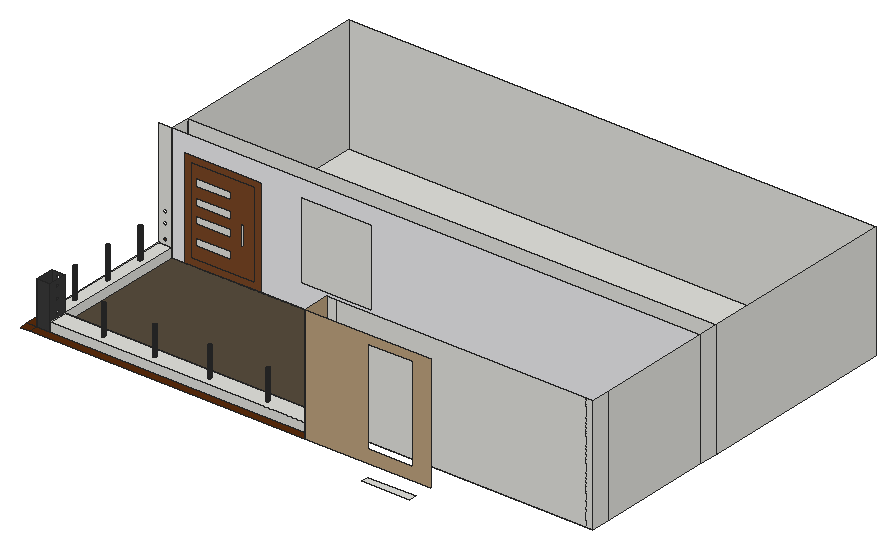
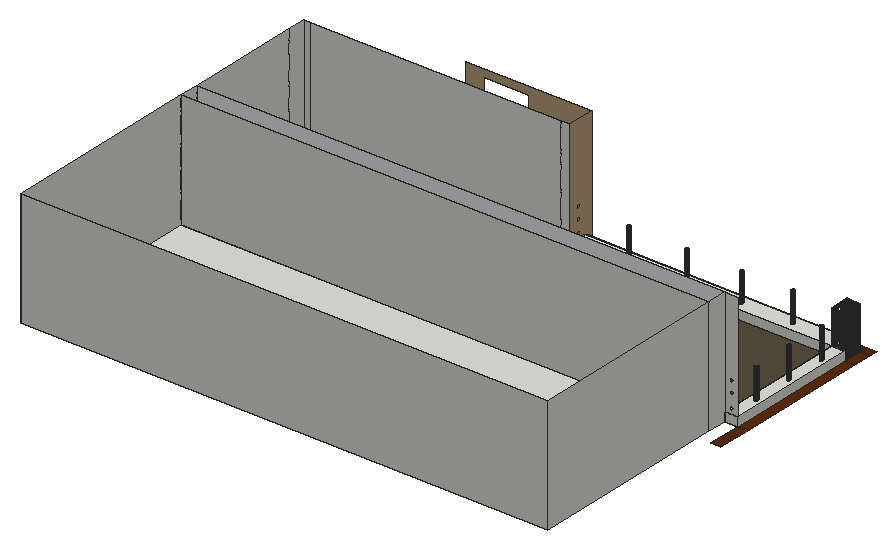
# SketchUp Ruby script. Lengths in inches.
U = 1.inch
M = Sketchup.active_model
def pt(a) = Geom::Point3d.new(a.map { |v| v * U })
def face(e, loops, mat)
  f = e.add_face(loops[0].map { |a| pt(a) })
  loops[1..].each { |l| e.add_face(l.map { |a| pt(a) }).erase! }
  f.material = f.back_material = mat if mat
  f
end
# faces: each face lists its corners as indices into pts; further lists are holes
def faces(e, pts, list, mat = nil) = list.each { |f| face(e, (f[0].is_a?(Array) ? f : [f]).map { |l| l.map { |i| pts[i] } }, mat) }
# xy, xz, yz: faces in a plane at the given z, y or x. An outline is a flat list of corners, or four numbers for a rectangle; further outlines are holes
def ring(l) = l.size == 4 ? [[l[0], l[1]], [l[2], l[1]], [l[2], l[3]], [l[0], l[3]]] : l.each_slice(2).to_a
def flat(e, list, mat, &to3) = list.each { |f| face(e, (f[0].is_a?(Array) ? f : [f]).map { |l| ring(l).map { |u, v| to3.(u, v) } }, mat) }
def xy(e, z, list, mat = nil) = flat(e, list, mat) { |x, y| [x, y, z] }
def xz(e, y, list, mat = nil) = flat(e, list, mat) { |x, z| [x, y, z] }
def yz(e, x, list, mat = nil) = flat(e, list, mat) { |y, z| [x, y, z] }
def lines(e, pts, list) = list.each { |a, b| e.add_line(pt(pts[a]), pt(pts[b])) }
# prism: a flat outline (further loops are holes) pulled along v
def prism(e, loops, v, mat = nil)
  f = face(e, loops, mat); d = Geom::Vector3d.new(v.map { |x| x * U })
  f.pushpull(f.normal.samedirection?(d) ? d.length : -d.length)
end
def box(e, o, s, mat = nil) = prism(e, [[o, [o[0] + s[0], o[1], o[2]], [o[0] + s[0], o[1] + s[1], o[2]], [o[0], o[1] + s[1], o[2]]]], [0, 0, s[2]], mat)
def at(x, y, z, deg = 0) = Geom::Transformation.translation(pt([x, y, z])) * Geom::Transformation.rotation(ORIGIN, Z_AXIS, deg.degrees)
def axes(o, x, y, z) = Geom::Transformation.new([*x, 0, *y, 0, *z, 0, *pt(o).to_a, 1])
def part(name) = M.definitions.add(name)
# library, detail: a bought-in or finely detailed component or shape, given as its bounding box
def library(name, o, s) = part(name).tap { |d| box(d.entities, o, s) }
def detail(e, o, s) = box(e.add_group.entities, o, s)
def put(e, d, t, mat = nil) = e.add_instance(d, t).tap { |i| i.material = mat if mat }
def group(e, t, mat = nil) = e.add_group.tap { |g| g.transformation = t; g.material = mat if mat }.entities
root = M.entities
M.materials.add("[0035_Tan]").color = [188, 161, 125]
M.materials.add("[0043_SaddleBrown]").color = [91, 44, 12]
M.materials.add("[Blinds Vertical Pattern]").color = [237, 237, 239]
M.materials.add("[Carpet Diamond Olive]").color = [87, 77, 61]
M.materials.add("[Color M07]").color = [58, 58, 58]
M.materials.add("[Wood Veneer 01]").color = [120, 70, 37]
xy(root,746.5625,[[378.18,386.34,421.12,393.34]])
xy(root,757.5,[[73.92,401.01,85.98,418.04],[85.98,401.01,320.99,418.04],[73.92,418.04,85.98,538.2],[85.98,538.2,560.26,556.28],[85.98,556.28,560.26,737.09]])
xy(root,757.5,[[65.42,393.34,73.92,401.01],[73.92,393.34,320.99,401.01],[65.42,401.01,73.92,418.04],[65.42,418.04,73.92,538.2],[65.42,538.2,73.92,568.32]],"[0043_SaddleBrown]")
xy(root,757.5,[[85.98,418.04,560.26,538.2]],"[Carpet Diamond Olive]")
xy(root,765.5625,[[[85.98,401.01,320.99,418.04],[127.44,407.81,127.05,407.86,126.69,408.01,126.38,408.25,126.14,408.56,125.99,408.92,125.94,409.31,125.99,409.7,126.14,410.06,126.38,410.37,126.69,410.61,127.05,410.76,127.44,410.81,127.83,410.76,128.19,410.61,128.5,410.37,128.74,410.06,128.89,409.7,128.94,409.31,128.89,408.92,128.74,408.56,128.5,408.25,128.19,408.01,127.83,407.86],[275.5,407.81,275.12,407.86,274.75,408.01,274.44,408.25,274.21,408.56,274.06,408.92,274,409.31,274.06,409.7,274.21,410.06,274.44,410.37,274.75,410.61,275.12,410.76,275.5,410.81,275.89,410.76,276.25,410.61,276.57,410.37,276.8,410.06,276.95,409.7,277,409.31,276.95,408.92,276.8,408.56,276.57,408.25,276.25,408.01,275.89,407.86],[173.82,407.81,173.43,407.86,173.07,408.01,172.76,408.25,172.52,408.56,172.37,408.92,172.32,409.31,172.37,409.7,172.52,410.06,172.76,410.37,173.07,410.61,173.43,410.76,173.82,410.81,174.21,410.76,174.57,410.61,174.88,410.37,175.12,410.06,175.27,409.7,175.32,409.31,175.27,408.92,175.12,408.56,174.88,408.25,174.57,408.01,174.21,407.86],[223,407.81,222.62,407.86,222.25,408.01,221.94,408.25,221.71,408.56,221.56,408.92,221.5,409.31,221.56,409.7,221.71,410.06,221.94,410.37,222.25,410.61,222.62,410.76,223,410.81,223.39,410.76,223.75,410.61,224.07,410.37,224.3,410.06,224.45,409.7,224.5,409.31,224.45,408.92,224.3,408.56,224.07,408.25,223.75,408.01,223.39,407.86]],[127.44,407.81,127.05,407.86,126.69,408.01,126.38,408.25,126.14,408.56,125.99,408.92,125.94,409.31,125.99,409.7,126.14,410.06,126.38,410.37,126.69,410.61,127.05,410.76,127.44,410.81,127.83,410.76,128.19,410.61,128.5,410.37,128.74,410.06,128.89,409.7,128.94,409.31,128.89,408.92,128.74,408.56,128.5,408.25,128.19,408.01,127.83,407.86],[173.82,407.81,173.43,407.86,173.07,408.01,172.76,408.25,172.52,408.56,172.37,408.92,172.32,409.31,172.37,409.7,172.52,410.06,172.76,410.37,173.07,410.61,173.43,410.76,173.82,410.81,174.21,410.76,174.57,410.61,174.88,410.37,175.12,410.06,175.27,409.7,175.32,409.31,175.27,408.92,175.12,408.56,174.88,408.25,174.57,408.01,174.21,407.86],[223,407.81,222.62,407.86,222.25,408.01,221.94,408.25,221.71,408.56,221.56,408.92,221.5,409.31,221.56,409.7,221.71,410.06,221.94,410.37,222.25,410.61,222.62,410.76,223,410.81,223.39,410.76,223.75,410.61,224.07,410.37,224.3,410.06,224.45,409.7,224.5,409.31,224.45,408.92,224.3,408.56,224.07,408.25,223.75,408.01,223.39,407.86],[275.5,407.81,275.12,407.86,274.75,408.01,274.44,408.25,274.21,408.56,274.06,408.92,274,409.31,274.06,409.7,274.21,410.06,274.44,410.37,274.75,410.61,275.12,410.76,275.5,410.81,275.89,410.76,276.25,410.61,276.57,410.37,276.8,410.06,276.95,409.7,277,409.31,276.95,408.92,276.8,408.56,276.57,408.25,276.25,408.01,275.89,407.86],
  [[73.92,418.04,85.98,538.2],[79.17,436.29,78.78,436.34,78.42,436.49,78.11,436.73,77.875,437.04,77.72,437.4,77.67,437.79,77.72,438.18,77.875,438.54,78.11,438.85,78.42,439.09,78.78,439.24,79.17,439.29,79.5625,439.24,79.92,439.09,80.23,438.85,80.47,438.54,80.62,438.18,80.67,437.79,80.62,437.4,80.47,437.04,80.23,436.73,79.92,436.49,79.5625,436.34],[79.17,509.6,78.78,509.65,78.42,509.8,78.11,510.04,77.875,510.35,77.72,510.71,77.67,511.1,77.72,511.49,77.875,511.85,78.11,512.16,78.42,512.4,78.78,512.55,79.17,512.6,79.5625,512.55,79.92,512.4,80.23,512.16,80.47,511.85,80.62,511.49,80.67,511.1,80.62,510.71,80.47,510.35,80.23,510.04,79.92,509.8,79.5625,509.65],[79.17,472.66,78.78,472.72,78.42,472.87,78.11,473.1,77.875,473.41,77.72,473.78,77.67,474.16,77.72,474.55,77.875,474.91,78.11,475.23,78.42,475.46,78.78,475.61,79.17,475.66,79.5625,475.61,79.92,475.46,80.23,475.23,80.47,474.91,80.62,474.55,80.67,474.16,80.62,473.78,80.47,473.41,80.23,473.1,79.92,472.87,79.5625,472.72]],[79.17,436.29,78.78,436.34,78.42,436.49,78.11,436.73,77.875,437.04,77.72,437.4,77.67,437.79,77.72,438.18,77.875,438.54,78.11,438.85,78.42,439.09,78.78,439.24,79.17,439.29,79.5625,439.24,79.92,439.09,80.23,438.85,80.47,438.54,80.62,438.18,80.67,437.79,80.62,437.4,80.47,437.04,80.23,436.73,79.92,436.49,79.5625,436.34],[79.17,472.66,78.78,472.72,78.42,472.87,78.11,473.1,77.875,473.41,77.72,473.78,77.67,474.16,77.72,474.55,77.875,474.91,78.11,475.23,78.42,475.46,78.78,475.61,79.17,475.66,79.5625,475.61,79.92,475.46,80.23,475.23,80.47,474.91,80.62,474.55,80.67,474.16,80.62,473.78,80.47,473.41,80.23,473.1,79.92,472.87,79.5625,472.72],[79.17,509.6,78.78,509.65,78.42,509.8,78.11,510.04,77.875,510.35,77.72,510.71,77.67,511.1,77.72,511.49,77.875,511.85,78.11,512.16,78.42,512.4,78.78,512.55,79.17,512.6,79.5625,512.55,79.92,512.4,80.23,512.16,80.47,511.85,80.62,511.49,80.67,511.1,80.62,510.71,80.47,510.35,80.23,510.04,79.92,509.8,79.5625,509.65]])
xz(root,393.34,[[[320.99,757.5,434.25,861.625],[378.07,769.18,418.25,854.55]]],"[0035_Tan]")
xz(root,401.01,[[85.98,757.5,320.99,765.5625]])
xz(root,401.01,[[73.92,757.5,85.98,796.5]],"[Color M07]")
xz(root,418.04,[[73.92,757.5,85.98,765.5625],[85.98,757.5,320.99,765.5625],[320.99,757.5,329.72,861.625],[329.72,757.5,554.62,861.625],[554.62,757.5,560.26,861.625]])
xz(root,418.04,[[[73.92,765.5625,85.98,796.5],[79.68,781.03,80.13,781.09,80.55,781.27,80.91,781.55,81.19,781.91,81.37,782.33,81.43,782.78,81.37,783.24,81.19,783.66,80.91,784.02,80.55,784.3,80.13,784.47,79.68,784.53,79.22,784.47,78.8,784.3,78.4375,784.02,78.16,783.66,77.99,783.24,77.93,782.78,77.99,782.33,78.16,781.91,78.4375,781.55,78.8,781.27,79.22,781.09],[79.68,768.35,80.13,768.41,80.55,768.58,80.91,768.86,81.19,769.22,81.37,769.64,81.43,770.1,81.37,770.55,81.19,770.97,80.91,771.33,80.55,771.61,80.13,771.79,79.68,771.85,79.22,771.79,78.8,771.61,78.4375,771.33,78.16,770.97,77.99,770.55,77.93,770.1,77.99,769.64,78.16,769.22,78.4375,768.86,78.8,768.58,79.22,768.41],[79.68,790.85,80.13,790.91,80.55,791.08,80.91,791.36,81.19,791.72,81.37,792.14,81.43,792.6,81.37,793.05,81.19,793.47,80.91,793.83,80.55,794.11,80.13,794.29,79.68,794.35,79.22,794.29,78.8,794.11,78.4375,793.83,78.16,793.47,77.99,793.05,77.93,792.6,77.99,792.14,78.16,791.72,78.4375,791.36,78.8,791.08,79.22,790.91]]],"[Color M07]")
xz(root,538.2,[[73.92,757.5,85.98,765.5625],[[73.92,765.5625,85.98,861.625],[79.68,768.35,79.22,768.41,78.8,768.58,78.4375,768.86,78.16,769.22,77.99,769.64,77.93,770.1,77.99,770.55,78.16,770.97,78.4375,771.33,78.8,771.61,79.22,771.79,79.68,771.85,80.13,771.79,80.55,771.61,80.91,771.33,81.19,770.97,81.37,770.55,81.43,770.1,81.37,769.64,81.19,769.22,80.91,768.86,80.55,768.58,80.13,768.41],[79.68,781.03,79.22,781.09,78.8,781.27,78.4375,781.55,78.16,781.91,77.99,782.33,77.93,782.78,77.99,783.24,78.16,783.66,78.4375,784.02,78.8,784.3,79.22,784.47,79.68,784.53,80.13,784.47,80.55,784.3,80.91,784.02,81.19,783.66,81.37,783.24,81.43,782.78,81.37,782.33,81.19,781.91,80.91,781.55,80.55,781.27,80.13,781.09],[79.68,790.85,79.22,790.91,78.8,791.08,78.4375,791.36,78.16,791.72,77.99,792.14,77.93,792.6,77.99,793.05,78.16,793.47,78.4375,793.83,78.8,794.11,79.22,794.29,79.68,794.35,80.13,794.29,80.55,794.11,80.91,793.83,81.19,793.47,81.37,793.05,81.43,792.6,81.37,792.14,81.19,791.72,80.91,791.36,80.55,791.08,80.13,790.91]]])
xz(root,538.2,[[[85.98,757.5,97.43,757.5,97.43,845.625,165.56,845.625,165.56,757.5,560.26,757.5,560.26,861.625,85.98,861.625],[201.38,777.72,265.3,846.97]]],"[Blinds Vertical Pattern]")
xz(root,538.2,[[[97.43,757.5,165.56,845.625],[102.8,762.87,160.18,840.25]],[[102.8,762.87,160.18,840.25],[107.76,822.27,138.82,829.34],[107.76,774.27,138.82,781.34],[107.76,806.52,138.82,813.59],[107.76,792.02,138.82,799.09],[147.39,788.3,150.51,806.24]]],"[Wood Veneer 01]")
xz(root,556.28,[[85.98,757.5,560.26,861.625]])
xz(root,737.09,[[85.98,757.5,560.26,861.625]])
yz(root,73.92,[[418.04,757.5,538.2,765.5625]])
yz(root,73.92,[[401.01,757.5,418.04,796.5]],"[Color M07]")
yz(root,85.98,[[401.01,757.5,418.04,765.5625],[418.04,757.5,538.2,765.5625],[538.2,757.5,556.28,861.625],[556.28,757.5,737.09,861.625]])
yz(root,85.98,[[[401.01,765.5625,418.04,796.5],[408.91,768.38,408.45,768.44,408.03,768.62,407.67,768.9,407.39,769.26,407.22,769.68,407.16,770.13,407.22,770.59,407.39,771.01,407.67,771.37,408.03,771.65,408.45,771.82,408.91,771.88,409.36,771.82,409.78,771.65,410.14,771.37,410.42,771.01,410.6,770.59,410.66,770.13,410.6,769.68,410.42,769.26,410.14,768.9,409.78,768.62,409.36,768.44],[408.91,789.82,408.45,789.88,408.03,790.06,407.67,790.33,407.39,790.7,407.22,791.12,407.16,791.57,407.22,792.02,407.39,792.45,407.67,792.81,408.03,793.09,408.45,793.26,408.91,793.32,409.36,793.26,409.78,793.09,410.14,792.81,410.42,792.45,410.6,792.02,410.66,791.57,410.6,791.12,410.42,790.7,410.14,790.33,409.78,790.06,409.36,789.88],[408.91,779.13,408.45,779.19,408.03,779.37,407.67,779.65,407.39,780.01,407.22,780.43,407.16,780.88,407.22,781.34,407.39,781.76,407.67,782.12,408.03,782.4,408.45,782.57,408.91,782.63,409.36,782.57,409.78,782.4,410.14,782.12,410.42,781.76,410.6,781.34,410.66,780.88,410.6,780.43,410.42,780.01,410.14,779.65,409.78,779.37,409.36,779.19]]],"[Color M07]")
yz(root,320.99,[[401.01,757.5,418.04,765.5625]])
yz(root,320.99,[[[393.34,757.5,393.34,861.625,418.04,861.625,418.04,765.5625,401.01,765.5625,401.01,757.5],[408.91,768.38,409.36,768.44,409.78,768.62,410.14,768.9,410.42,769.26,410.6,769.68,410.66,770.13,410.6,770.59,410.42,771.01,410.14,771.37,409.78,771.65,409.36,771.82,408.91,771.88,408.45,771.82,408.03,771.65,407.67,771.37,407.39,771.01,407.22,770.59,407.16,770.13,407.22,769.68,407.39,769.26,407.67,768.9,408.03,768.62,408.45,768.44],[408.91,789.82,409.36,789.88,409.78,790.06,410.14,790.33,410.42,790.7,410.6,791.12,410.66,791.57,410.6,792.02,410.42,792.45,410.14,792.81,409.78,793.09,409.36,793.26,408.91,793.32,408.45,793.26,408.03,793.09,407.67,792.81,407.39,792.45,407.22,792.02,407.16,791.57,407.22,791.12,407.39,790.7,407.67,790.33,408.03,790.06,408.45,789.88],[408.91,779.13,409.36,779.19,409.78,779.37,410.14,779.65,410.42,780.01,410.6,780.43,410.66,780.88,410.6,781.34,410.42,781.76,410.14,782.12,409.78,782.4,409.36,782.57,408.91,782.63,408.45,782.57,408.03,782.4,407.67,782.12,407.39,781.76,407.22,781.34,407.16,780.88,407.22,780.43,407.39,780.01,407.67,779.65,408.03,779.37,408.45,779.19]]],"[0035_Tan]")
yz(root,560.26,[[418.04,757.5,434.85,861.625],[434.85,757.5,538.2,861.625],[538.2,757.5,556.28,861.625],[556.28,757.5,737.09,861.625]])
p = [[127.05,407.86,765.5625],[127.44,407.81,765.5625],[127.44,407.81,792.02],[127.05,407.86,792.02],[127.83,407.86,765.5625],[127.83,407.86,792.02],
  [173.43,407.86,765.5625],[173.82,407.81,765.5625],[173.82,407.81,791.0625],[173.43,407.86,791.0625],[174.21,407.86,765.5625],[174.21,407.86,791.0625],
  [222.62,407.86,765.5625],[223,407.81,765.5625],[223,407.81,791.57],[222.62,407.86,791.57],[223.39,407.86,765.5625],[223.39,407.86,791.57],
  [275.12,407.86,765.5625],[275.5,407.81,765.5625],[275.5,407.81,791.5625],[275.12,407.86,791.5625],[275.89,407.86,765.5625],[275.89,407.86,791.5625],
  [126.69,408.01,765.5625],[126.69,408.01,792.02],[128.19,408.01,765.5625],[128.19,408.01,792.02],[173.07,408.01,765.5625],[173.07,408.01,791.0625],
  [174.57,408.01,765.5625],[174.57,408.01,791.0625],[222.25,408.01,765.5625],[222.25,408.01,791.57],[223.75,408.01,765.5625],[223.75,408.01,791.57],
  [274.75,408.01,765.5625],[274.75,408.01,791.5625],[276.25,408.01,765.5625],[276.25,408.01,791.5625],[126.38,408.25,765.5625],[126.38,408.25,792.02],
  [128.5,408.25,765.5625],[128.5,408.25,792.02],[172.76,408.25,765.5625],[172.76,408.25,791.0625],[174.88,408.25,765.5625],[174.88,408.25,791.0625],
  [221.94,408.25,765.5625],[221.94,408.25,791.57],[224.07,408.25,765.5625],[224.07,408.25,791.57],[274.44,408.25,765.5625],[274.44,408.25,791.5625],
  [276.57,408.25,765.5625],[276.57,408.25,791.5625],[126.14,408.56,765.5625],[126.14,408.56,792.02],[128.74,408.56,765.5625],[128.74,408.56,792.02],
  [172.52,408.56,765.5625],[172.52,408.56,791.0625],[175.12,408.56,765.5625],[175.12,408.56,791.0625],[221.71,408.56,765.5625],[221.71,408.56,791.57],
  [224.3,408.56,765.5625],[224.3,408.56,791.57],[274.21,408.56,765.5625],[274.21,408.56,791.5625],[276.8,408.56,765.5625],[276.8,408.56,791.5625],
  [125.99,408.92,765.5625],[125.99,408.92,792.02],[128.89,408.92,765.5625],[128.89,408.92,792.02],[172.37,408.92,765.5625],[172.37,408.92,791.0625],
  [175.27,408.92,765.5625],[175.27,408.92,791.0625],[221.56,408.92,765.5625],[221.56,408.92,791.57],[224.45,408.92,765.5625],[224.45,408.92,791.57],
  [274.06,408.92,765.5625],[274.06,408.92,791.5625],[276.95,408.92,765.5625],[276.95,408.92,791.5625],[125.94,409.31,765.5625],[125.94,409.31,792.02],
  [128.94,409.31,765.5625],[128.94,409.31,792.02],[172.32,409.31,765.5625],[172.32,409.31,791.0625],[175.32,409.31,765.5625],[175.32,409.31,791.0625],
  [221.5,409.31,765.5625],[221.5,409.31,791.57],[224.5,409.31,765.5625],[224.5,409.31,791.57],[274,409.31,765.5625],[274,409.31,791.5625],
  [277,409.31,765.5625],[277,409.31,791.5625],[125.99,409.7,765.5625],[125.99,409.7,792.02],[128.89,409.7,765.5625],[128.89,409.7,792.02],
  [172.37,409.7,765.5625],[172.37,409.7,791.0625],[175.27,409.7,765.5625],[175.27,409.7,791.0625],[221.56,409.7,765.5625],[221.56,409.7,791.57],
  [224.45,409.7,765.5625],[224.45,409.7,791.57],[274.06,409.7,765.5625],[274.06,409.7,791.5625],[276.95,409.7,765.5625],[276.95,409.7,791.5625],
  [126.14,410.06,765.5625],[126.14,410.06,792.02],[128.74,410.06,765.5625],[128.74,410.06,792.02],[172.52,410.06,765.5625],[172.52,410.06,791.0625],
  [175.12,410.06,765.5625],[175.12,410.06,791.0625],[221.71,410.06,765.5625],[221.71,410.06,791.57],[224.3,410.06,765.5625],[224.3,410.06,791.57],
  [274.21,410.06,765.5625],[274.21,410.06,791.5625],[276.8,410.06,765.5625],[276.8,410.06,791.5625],[126.38,410.37,765.5625],[126.38,410.37,792.02],
  [128.5,410.37,765.5625],[128.5,410.37,792.02],[172.76,410.37,765.5625],[172.76,410.37,791.0625],[174.88,410.37,765.5625],[174.88,410.37,791.0625],
  [221.94,410.37,765.5625],[221.94,410.37,791.57],[224.07,410.37,765.5625],[224.07,410.37,791.57],[274.44,410.37,765.5625],[274.44,410.37,791.5625],
  [276.57,410.37,765.5625],[276.57,410.37,791.5625],[126.69,410.61,765.5625],[126.68,410.6,792.02],[126.69,410.61,792.02],[128.19,410.61,765.5625],
  [128.19,410.61,792.02],[128.2,410.6,792.02],[173.07,410.61,765.5625],[173.07,410.61,791.0625],[174.57,410.61,765.5625],[174.57,410.61,791.0625],
  [222.25,410.61,765.5625],[222.25,410.61,791.57],[223.75,410.61,765.5625],[223.75,410.61,791.57],[274.75,410.61,765.5625],[274.75,410.61,791.5625],
  [276.25,410.61,765.5625],[276.25,410.61,791.5625],[127.05,410.76,765.5625],[127.05,410.76,792.02],[127.83,410.76,765.5625],[127.83,410.76,792.02],
  [173.43,410.76,765.5625],[173.43,410.76,791.0625],[174.21,410.76,765.5625],[174.21,410.76,791.0625],[222.62,410.76,765.5625],[222.38,410.66,791.57],
  [222.62,410.76,791.57],[223.39,410.76,765.5625],[223.39,410.76,791.57],[223.63,410.66,791.57],[275.12,410.76,765.5625],[275.12,410.76,791.5625],
  [275.89,410.76,765.5625],[275.89,410.76,791.5625],[127.44,410.81,765.5625],[127.44,410.81,792.02],[173.82,410.81,765.5625],[173.82,410.81,791.0625],
  [223,410.81,765.5625],[223,410.81,791.57],[275.5,410.81,765.5625],[275.5,410.81,791.5625],[78.42,436.49,765.5625],[78.78,436.34,765.5625],
  [78.78,436.34,792.5625],[78.42,436.49,792.5625],[79.17,436.29,765.5625],[79.17,436.29,792.5625],[79.5625,436.34,765.5625],[79.5625,436.34,792.5625],
  [79.92,436.49,765.5625],[79.92,436.49,792.5625],[78.11,436.73,765.5625],[78.11,436.73,792.5625],[80.23,436.73,765.5625],[80.23,436.73,792.5625],
  [77.875,437.04,765.5625],[77.875,437.04,792.5625],[80.47,437.04,765.5625],[80.47,437.04,792.5625],[77.72,437.4,765.5625],[77.72,437.4,792.5625],
  [80.62,437.4,765.5625],[80.62,437.4,792.5625],[77.67,437.79,765.5625],[77.67,437.79,792.5625],[80.67,437.79,765.5625],[80.67,437.79,792.5625],
  [77.72,438.18,765.5625],[77.72,438.18,792.5625],[80.62,438.18,765.5625],[80.62,438.18,792.5625],[77.875,438.54,765.5625],[77.875,438.54,792.5625],
  [80.47,438.54,765.5625],[80.47,438.54,792.5625],[78.11,438.85,765.5625],[78.11,438.85,792.5625],[80.23,438.85,765.5625],[80.23,438.85,792.5625],
  [78.42,439.09,765.5625],[78.42,439.09,792.5625],[79.92,439.09,765.5625],[79.92,439.09,792.5625],[78.78,439.24,765.5625],[78.78,439.24,792.5625],
  [79.5625,439.24,765.5625],[79.5625,439.24,792.5625],[79.17,439.29,765.5625],[79.17,439.29,792.5625],[78.42,472.87,765.5625],[78.78,472.72,765.5625],
  [78.78,472.72,793.125],[78.42,472.87,793.125],[79.17,472.66,765.5625],[79.17,472.66,793.125],[79.5625,472.72,765.5625],[79.5625,472.72,793.125],
  [79.92,472.87,765.5625],[79.92,472.87,793.125],[78.11,473.1,765.5625],[78.11,473.1,793.125],[80.23,473.1,765.5625],[80.23,473.1,793.125],
  [77.875,473.41,765.5625],[77.875,473.41,793.125],[80.47,473.41,765.5625],[80.47,473.41,793.125],[77.72,473.78,765.5625],[77.72,473.78,793.125],
  [80.62,473.78,765.5625],[80.62,473.78,793.125],[77.67,474.16,765.5625],[77.67,474.16,793.125],[80.67,474.16,765.5625],[80.67,474.16,793.125],
  [77.72,474.55,765.5625],[77.72,474.55,793.125],[80.62,474.55,765.5625],[80.62,474.55,793.125],[77.875,474.91,765.5625],[77.875,474.91,793.125],
  [80.47,474.91,765.5625],[80.47,474.91,793.125],[78.11,475.23,765.5625],[78.11,475.23,793.125],[80.23,475.23,765.5625],[80.23,475.23,793.125],
  [78.42,475.46,765.5625],[78.42,475.46,793.125],[79.92,475.46,765.5625],[79.92,475.46,793.125],[78.78,475.61,765.5625],[78.78,475.61,793.125],
  [79.5625,475.61,765.5625],[79.5625,475.61,793.125],[79.17,475.66,765.5625],[79.17,475.66,793.125],[78.78,509.65,765.5625],[79.17,509.6,765.5625],
  [79.17,509.6,792.3125],[78.78,509.65,792.3125],[79.5625,509.65,765.5625],[79.5625,509.65,792.3125],[78.42,509.8,765.5625],[78.42,509.8,792.3125],
  [79.92,509.8,765.5625],[79.92,509.8,792.3125],[78.11,510.04,765.5625],[78.11,510.04,792.3125],[80.23,510.04,765.5625],[80.23,510.04,792.3125],
  [77.875,510.35,765.5625],[77.875,510.35,792.3125],[80.47,510.35,765.5625],[80.47,510.35,792.3125],[77.72,510.71,765.5625],[77.72,510.71,792.3125],
  [80.62,510.71,765.5625],[80.62,510.71,792.3125],[77.67,511.1,765.5625],[77.67,511.1,792.3125],[80.67,511.1,765.5625],[80.67,511.1,792.3125],
  [77.72,511.49,765.5625],[77.72,511.49,792.3125],[80.62,511.49,765.5625],[80.62,511.49,792.3125],[77.875,511.85,765.5625],[77.875,511.85,792.3125],
  [80.47,511.85,765.5625],[80.47,511.85,792.3125],[78.11,512.16,765.5625],[78.11,512.16,792.3125],[80.23,512.16,765.5625],[80.23,512.16,792.3125],
  [78.42,512.4,765.5625],[78.42,512.4,792.3125],[79.92,512.4,765.5625],[79.92,512.4,792.3125],[78.78,512.55,765.5625],[78.78,512.55,792.3125],
  [79.5625,512.55,765.5625],[79.5625,512.55,792.3125],[79.17,512.6,765.5625],[79.17,512.6,792.3125]]
faces(root,p,[[0,1,2,3],[1,4,5,2],[6,7,8,9],[7,10,11,8],[12,13,14,15],[13,16,17,14],[18,19,20,21],[19,22,23,20],
  [24,0,3,25],[4,26,27,5],[28,6,9,29],[10,30,31,11],[32,12,15,33],[16,34,35,17],[36,18,21,37],[22,38,39,23],
  [40,24,25,41],[26,42,43,27],[44,28,29,45],[30,46,47,31],[48,32,33,49],[34,50,51,35],[52,36,37,53],[38,54,55,39],
  [56,40,41,57],[42,58,59,43],[60,44,45,61],[46,62,63,47],[64,48,49,65],[50,66,67,51],[68,52,53,69],[54,70,71,55],
  [72,56,57,73],[58,74,75,59],[76,60,61,77],[62,78,79,63],[80,64,65,81],[66,82,83,67],[84,68,69,85],[70,86,87,71],
  [88,72,73,89],[74,90,91,75],[92,76,77,93],[78,94,95,79],[96,80,81,97],[82,98,99,83],[100,84,85,101],[86,102,103,87],
  [104,88,89,105],[90,106,107,91],[108,92,93,109],[94,110,111,95],[112,96,97,113],[98,114,115,99],[116,100,101,117],[102,118,119,103],
  [120,104,105,121],[106,122,123,107],[124,108,109,125],[110,126,127,111],[128,112,113,129],[114,130,131,115],[132,116,117,133],[118,134,135,119],
  [136,120,121,137],[122,138,139,123],[140,124,125,141],[126,142,143,127],[144,128,129,145],[130,146,147,131],[148,132,133,149],[134,150,151,135],
  [152,136,137,153,154],[138,155,156,157,139],[158,140,141,159],[142,160,161,143],[162,144,145,163],[146,164,165,147],[166,148,149,167],[150,168,169,151],
  [170,152,154,171],[155,172,173,156],[174,158,159,175],[160,176,177,161],[178,162,163,179,180],[164,181,182,183,165],[184,166,167,185],[168,186,187,169],
  [188,170,171,189],[172,188,189,173],[190,174,175,191],[176,190,191,177],[192,178,180,193],[181,192,193,182],[194,184,185,195],[186,194,195,187],
  [196,197,198,199],[197,200,201,198],[200,202,203,201],[202,204,205,203],[206,196,199,207],[204,208,209,205],[210,206,207,211],[208,212,213,209],
  [214,210,211,215],[212,216,217,213],[218,214,215,219],[216,220,221,217],[222,218,219,223],[220,224,225,221],[226,222,223,227],[224,228,229,225],
  [230,226,227,231],[228,232,233,229],[234,230,231,235],[232,236,237,233],[238,234,235,239],[236,240,241,237],[242,238,239,243],[240,242,243,241],
  [244,245,246,247],[245,248,249,246],[248,250,251,249],[250,252,253,251],[254,244,247,255],[252,256,257,253],[258,254,255,259],[256,260,261,257],
  [262,258,259,263],[260,264,265,261],[266,262,263,267],[264,268,269,265],[270,266,267,271],[268,272,273,269],[274,270,271,275],[272,276,277,273],
  [278,274,275,279],[276,280,281,277],[282,278,279,283],[280,284,285,281],[286,282,283,287],[284,288,289,285],[290,286,287,291],[288,290,291,289],
  [292,293,294,295],[293,296,297,294],[298,292,295,299],[296,300,301,297],[302,298,299,303],[300,304,305,301],[306,302,303,307],[304,308,309,305],
  [310,306,307,311],[308,312,313,309],[314,310,311,315],[312,316,317,313],[318,314,315,319],[316,320,321,317],[322,318,319,323],[320,324,325,321],
  [326,322,323,327],[324,328,329,325],[330,326,327,331],[328,332,333,329],[334,330,331,335],[332,336,337,333],[338,334,335,339],[336,338,339,337]],"[Color M07]")
